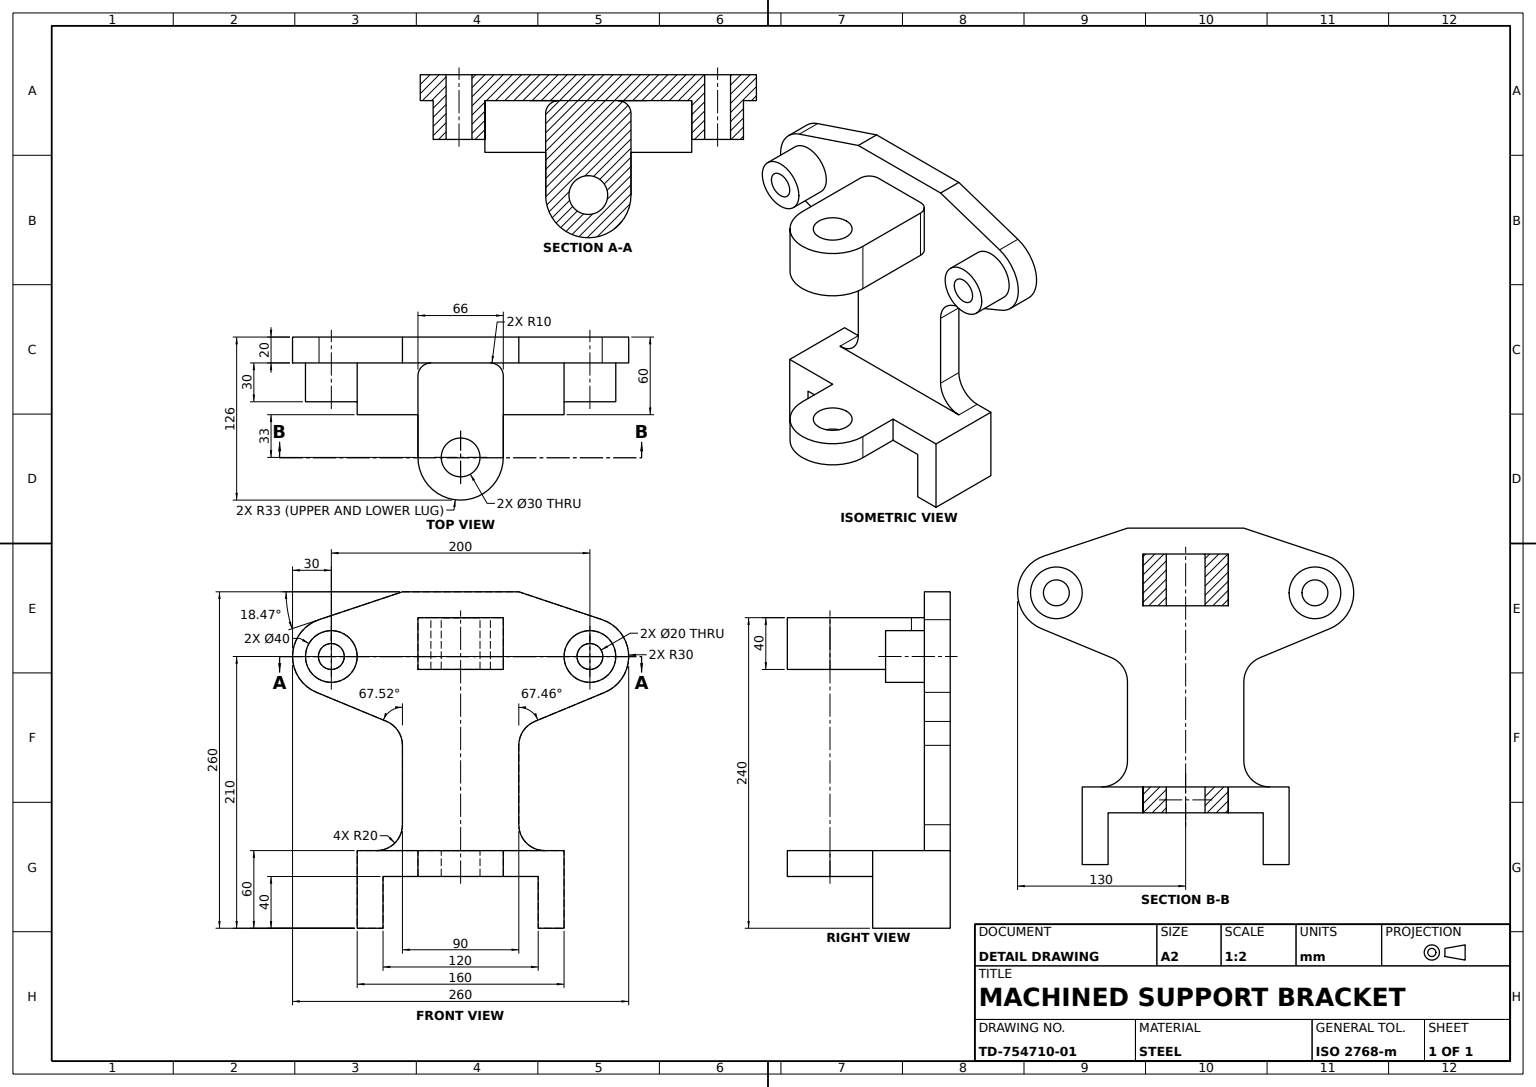
ISO-10303-21;
HEADER;
FILE_DESCRIPTION((''),'2;1');
FILE_NAME('','',(''),(''),'','','');
FILE_SCHEMA(('AUTOMOTIVE_DESIGN'));
ENDSEC;
DATA;
#1=APPLICATION_CONTEXT('');
#2=PRODUCT_CONTEXT('',#1,'mechanical');
#3=PRODUCT('','','',(#2));
#4=PRODUCT_DEFINITION_FORMATION('','',#3);
#5=PRODUCT_DEFINITION_CONTEXT('',#1,'design');
#6=PRODUCT_DEFINITION('','',#4,#5);
#7=PRODUCT_DEFINITION_SHAPE('','',#6);
#8=(LENGTH_UNIT()NAMED_UNIT(*)SI_UNIT(.MILLI.,.METRE.));
#9=(NAMED_UNIT(*)PLANE_ANGLE_UNIT()SI_UNIT($,.RADIAN.));
#10=(NAMED_UNIT(*)SI_UNIT($,.STERADIAN.)SOLID_ANGLE_UNIT());
#11=UNCERTAINTY_MEASURE_WITH_UNIT(LENGTH_MEASURE(1.E-05),#8,'distance_accuracy_value','');
#12=(GEOMETRIC_REPRESENTATION_CONTEXT(3)GLOBAL_UNCERTAINTY_ASSIGNED_CONTEXT((#11))GLOBAL_UNIT_ASSIGNED_CONTEXT((#8,#9,#10))REPRESENTATION_CONTEXT('',''));
#13=CARTESIAN_POINT('',(125.,260.,0.));
#14=VERTEX_POINT('',#13);
#15=CARTESIAN_POINT('',(35.,260.,0.));
#16=VERTEX_POINT('',#15);
#17=DIRECTION('',(-1.,0.,0.));
#18=VECTOR('',#17,1000.);
#19=LINE('',#15,#18);
#20=EDGE_CURVE('',#14,#16,#19,.T.);
#21=ORIENTED_EDGE('',*,*,#20,.T.);
#22=CARTESIAN_POINT('',(35.,260.,20.));
#23=VERTEX_POINT('',#22);
#24=DIRECTION('',(0.,0.,-1.));
#25=VECTOR('',#24,1000.);
#26=LINE('',#22,#25);
#27=EDGE_CURVE('',#23,#16,#26,.T.);
#28=ORIENTED_EDGE('',*,*,#27,.F.);
#29=CARTESIAN_POINT('',(125.,260.,20.));
#30=VERTEX_POINT('',#29);
#31=LINE('',#22,#18);
#32=EDGE_CURVE('',#30,#23,#31,.T.);
#33=ORIENTED_EDGE('',*,*,#32,.F.);
#34=LINE('',#29,#25);
#35=EDGE_CURVE('',#30,#14,#34,.T.);
#36=ORIENTED_EDGE('',*,*,#35,.T.);
#37=EDGE_LOOP('',(#21,#28,#33,#36));
#38=FACE_OUTER_BOUND('',#37,.T.);
#39=DIRECTION('',(0.,-1.,0.));
#40=AXIS2_PLACEMENT_3D('',#22,#39,#24);
#41=PLANE('',#40);
#42=ADVANCED_FACE('',(#38),#41,.F.);
#43=CARTESIAN_POINT('',(0.,60.,0.));
#44=VERTEX_POINT('',#43);
#45=CARTESIAN_POINT('',(0.,0.,0.));
#46=VERTEX_POINT('',#45);
#47=VECTOR('',#39,1000.);
#48=LINE('',#45,#47);
#49=EDGE_CURVE('',#44,#46,#48,.T.);
#50=ORIENTED_EDGE('',*,*,#49,.T.);
#51=CARTESIAN_POINT('',(0.,0.,60.));
#52=VERTEX_POINT('',#51);
#53=LINE('',#51,#25);
#54=EDGE_CURVE('',#52,#46,#53,.T.);
#55=ORIENTED_EDGE('',*,*,#54,.F.);
#56=CARTESIAN_POINT('',(0.,60.,60.));
#57=VERTEX_POINT('',#56);
#58=LINE('',#51,#47);
#59=EDGE_CURVE('',#57,#52,#58,.T.);
#60=ORIENTED_EDGE('',*,*,#59,.F.);
#61=LINE('',#56,#25);
#62=EDGE_CURVE('',#57,#44,#61,.T.);
#63=ORIENTED_EDGE('',*,*,#62,.T.);
#64=EDGE_LOOP('',(#50,#55,#60,#63));
#65=FACE_OUTER_BOUND('',#64,.T.);
#66=DIRECTION('',(1.,0.,0.));
#67=AXIS2_PLACEMENT_3D('',#51,#66,#24);
#68=PLANE('',#67);
#69=ADVANCED_FACE('',(#65),#68,.F.);
#70=CARTESIAN_POINT('',(170.,210.,50.));
#71=VERTEX_POINT('',#70);
#72=CARTESIAN_POINT('',(170.,210.,0.));
#73=VERTEX_POINT('',#72);
#74=LINE('',#70,#25);
#75=EDGE_CURVE('',#71,#73,#74,.T.);
#76=ORIENTED_EDGE('',*,*,#75,.T.);
#77=CARTESIAN_POINT('',(190.,210.,0.));
#78=VERTEX_POINT('',#77);
#79=CARTESIAN_POINT('',(180.,210.,0.));
#80=AXIS2_PLACEMENT_3D('',#79,#24,#17);
#81=CIRCLE('',#80,10.);
#82=EDGE_CURVE('',#73,#78,#81,.T.);
#83=ORIENTED_EDGE('',*,*,#82,.T.);
#84=CARTESIAN_POINT('',(190.,210.,50.));
#85=VERTEX_POINT('',#84);
#86=LINE('',#84,#25);
#87=EDGE_CURVE('',#85,#78,#86,.T.);
#88=ORIENTED_EDGE('',*,*,#87,.F.);
#89=CARTESIAN_POINT('',(180.,210.,50.));
#90=DIRECTION('',(0.,0.,1.));
#91=AXIS2_PLACEMENT_3D('',#89,#90,#66);
#92=CIRCLE('',#91,10.);
#93=EDGE_CURVE('',#85,#71,#92,.T.);
#94=ORIENTED_EDGE('',*,*,#93,.T.);
#95=EDGE_LOOP('',(#76,#83,#88,#94));
#96=FACE_OUTER_BOUND('',#95,.T.);
#97=AXIS2_PLACEMENT_3D('',#89,#24,#17);
#98=CYLINDRICAL_SURFACE('',#97,10.);
#99=ADVANCED_FACE('',(#96),#98,.F.);
#100=CARTESIAN_POINT('',(47.,60.,60.));
#101=VERTEX_POINT('',#100);
#102=CARTESIAN_POINT('',(47.,60.,93.));
#103=VERTEX_POINT('',#102);
#104=VECTOR('',#90,1000.);
#105=LINE('',#102,#104);
#106=EDGE_CURVE('',#101,#103,#105,.T.);
#107=ORIENTED_EDGE('',*,*,#106,.F.);
#108=CARTESIAN_POINT('',(47.,40.,60.));
#109=VERTEX_POINT('',#108);
#110=DIRECTION('',(0.,1.,0.));
#111=VECTOR('',#110,1000.);
#112=LINE('',#108,#111);
#113=EDGE_CURVE('',#109,#101,#112,.T.);
#114=ORIENTED_EDGE('',*,*,#113,.F.);
#115=CARTESIAN_POINT('',(47.,40.,93.));
#116=VERTEX_POINT('',#115);
#117=LINE('',#115,#104);
#118=EDGE_CURVE('',#109,#116,#117,.T.);
#119=ORIENTED_EDGE('',*,*,#118,.T.);
#120=LINE('',#115,#111);
#121=EDGE_CURVE('',#116,#103,#120,.T.);
#122=ORIENTED_EDGE('',*,*,#121,.T.);
#123=EDGE_LOOP('',(#107,#114,#119,#122));
#124=FACE_OUTER_BOUND('',#123,.T.);
#125=AXIS2_PLACEMENT_3D('',#115,#17,#90);
#126=PLANE('',#125);
#127=ADVANCED_FACE('',(#124),#126,.T.);
#128=CARTESIAN_POINT('',(80.,200.,108.));
#129=VERTEX_POINT('',#128);
#130=CARTESIAN_POINT('',(80.,200.,78.));
#131=VERTEX_POINT('',#130);
#132=CARTESIAN_POINT('',(80.,200.,93.));
#133=AXIS2_PLACEMENT_3D('',#132,#110,#90);
#134=CIRCLE('',#133,15.);
#135=EDGE_CURVE('',#129,#131,#134,.T.);
#136=ORIENTED_EDGE('',*,*,#135,.F.);
#137=CARTESIAN_POINT('',(80.,240.,108.));
#138=VERTEX_POINT('',#137);
#139=LINE('',#128,#111);
#140=EDGE_CURVE('',#129,#138,#139,.T.);
#141=ORIENTED_EDGE('',*,*,#140,.T.);
#142=CARTESIAN_POINT('',(80.,240.,78.));
#143=VERTEX_POINT('',#142);
#144=CARTESIAN_POINT('',(80.,240.,93.));
#145=AXIS2_PLACEMENT_3D('',#144,#110,#90);
#146=CIRCLE('',#145,15.);
#147=EDGE_CURVE('',#138,#143,#146,.T.);
#148=ORIENTED_EDGE('',*,*,#147,.T.);
#149=LINE('',#130,#111);
#150=EDGE_CURVE('',#131,#143,#149,.T.);
#151=ORIENTED_EDGE('',*,*,#150,.F.);
#152=EDGE_LOOP('',(#136,#141,#148,#151));
#153=FACE_OUTER_BOUND('',#152,.T.);
#154=CYLINDRICAL_SURFACE('',#133,15.);
#155=ADVANCED_FACE('',(#153),#154,.F.);
#156=CARTESIAN_POINT('',(80.,60.,78.));
#157=VERTEX_POINT('',#156);
#158=CARTESIAN_POINT('',(80.,60.,108.));
#159=VERTEX_POINT('',#158);
#160=CARTESIAN_POINT('',(80.,60.,93.));
#161=AXIS2_PLACEMENT_3D('',#160,#110,#90);
#162=CIRCLE('',#161,15.);
#163=EDGE_CURVE('',#157,#159,#162,.T.);
#164=ORIENTED_EDGE('',*,*,#163,.T.);
#165=CARTESIAN_POINT('',(80.,40.,108.));
#166=VERTEX_POINT('',#165);
#167=LINE('',#165,#111);
#168=EDGE_CURVE('',#166,#159,#167,.T.);
#169=ORIENTED_EDGE('',*,*,#168,.F.);
#170=CARTESIAN_POINT('',(80.,40.,78.));
#171=VERTEX_POINT('',#170);
#172=CARTESIAN_POINT('',(80.,40.,93.));
#173=AXIS2_PLACEMENT_3D('',#172,#110,#90);
#174=CIRCLE('',#173,15.);
#175=EDGE_CURVE('',#171,#166,#174,.T.);
#176=ORIENTED_EDGE('',*,*,#175,.F.);
#177=LINE('',#170,#111);
#178=EDGE_CURVE('',#171,#157,#177,.T.);
#179=ORIENTED_EDGE('',*,*,#178,.T.);
#180=EDGE_LOOP('',(#164,#169,#176,#179));
#181=FACE_OUTER_BOUND('',#180,.T.);
#182=CYLINDRICAL_SURFACE('',#173,15.);
#183=ADVANCED_FACE('',(#181),#182,.F.);
#184=CARTESIAN_POINT('',(22.646832,159.886795,20.));
#185=VERTEX_POINT('',#184);
#186=CARTESIAN_POINT('',(22.646832,159.886795,0.));
#187=VERTEX_POINT('',#186);
#188=LINE('',#184,#25);
#189=EDGE_CURVE('',#185,#187,#188,.T.);
#190=ORIENTED_EDGE('',*,*,#189,.T.);
#191=CARTESIAN_POINT('',(35.,141.406374,0.));
#192=VERTEX_POINT('',#191);
#193=CARTESIAN_POINT('',(15.,141.406374,0.));
#194=AXIS2_PLACEMENT_3D('',#193,#24,#66);
#195=CIRCLE('',#194,20.);
#196=EDGE_CURVE('',#187,#192,#195,.T.);
#197=ORIENTED_EDGE('',*,*,#196,.T.);
#198=CARTESIAN_POINT('',(35.,141.406374,20.));
#199=VERTEX_POINT('',#198);
#200=LINE('',#198,#25);
#201=EDGE_CURVE('',#199,#192,#200,.T.);
#202=ORIENTED_EDGE('',*,*,#201,.F.);
#203=CARTESIAN_POINT('',(15.,141.406374,20.));
#204=AXIS2_PLACEMENT_3D('',#203,#24,#66);
#205=CIRCLE('',#204,20.);
#206=EDGE_CURVE('',#185,#199,#205,.T.);
#207=ORIENTED_EDGE('',*,*,#206,.F.);
#208=EDGE_LOOP('',(#190,#197,#202,#207));
#209=FACE_OUTER_BOUND('',#208,.T.);
#210=AXIS2_PLACEMENT_3D('',#203,#24,#17);
#211=CYLINDRICAL_SURFACE('',#210,20.);
#212=ADVANCED_FACE('',(#209),#211,.F.);
#213=CARTESIAN_POINT('',(-29.504259,238.454684,20.));
#214=VERTEX_POINT('',#213);
#215=CARTESIAN_POINT('',(-29.504259,238.454684,0.));
#216=VERTEX_POINT('',#215);
#217=LINE('',#213,#25);
#218=EDGE_CURVE('',#214,#216,#217,.T.);
#219=ORIENTED_EDGE('',*,*,#218,.F.);
#220=DIRECTION('',(-0.948489482,-0.31680862,0.));
#221=VECTOR('',#220,1000.);
#222=LINE('',#22,#221);
#223=EDGE_CURVE('',#23,#214,#222,.T.);
#224=ORIENTED_EDGE('',*,*,#223,.F.);
#225=ORIENTED_EDGE('',*,*,#27,.T.);
#226=LINE('',#15,#221);
#227=EDGE_CURVE('',#16,#216,#226,.T.);
#228=ORIENTED_EDGE('',*,*,#227,.T.);
#229=EDGE_LOOP('',(#219,#224,#225,#228));
#230=FACE_OUTER_BOUND('',#229,.T.);
#231=DIRECTION('',(0.31680862,-0.948489482,0.));
#232=DIRECTION('',(0.948489482,0.31680862,0.));
#233=AXIS2_PLACEMENT_3D('',#22,#231,#232);
#234=PLANE('',#233);
#235=ADVANCED_FACE('',(#230),#234,.F.);
#236=CARTESIAN_POINT('',(160.,0.,0.));
#237=VERTEX_POINT('',#236);
#238=CARTESIAN_POINT('',(160.,60.,0.));
#239=VERTEX_POINT('',#238);
#240=LINE('',#238,#111);
#241=EDGE_CURVE('',#237,#239,#240,.T.);
#242=ORIENTED_EDGE('',*,*,#241,.T.);
#243=CARTESIAN_POINT('',(160.,60.,60.));
#244=VERTEX_POINT('',#243);
#245=LINE('',#243,#25);
#246=EDGE_CURVE('',#244,#239,#245,.T.);
#247=ORIENTED_EDGE('',*,*,#246,.F.);
#248=CARTESIAN_POINT('',(160.,0.,60.));
#249=VERTEX_POINT('',#248);
#250=LINE('',#243,#111);
#251=EDGE_CURVE('',#249,#244,#250,.T.);
#252=ORIENTED_EDGE('',*,*,#251,.F.);
#253=LINE('',#248,#25);
#254=EDGE_CURVE('',#249,#237,#253,.T.);
#255=ORIENTED_EDGE('',*,*,#254,.T.);
#256=EDGE_LOOP('',(#242,#247,#252,#255));
#257=FACE_OUTER_BOUND('',#256,.T.);
#258=AXIS2_PLACEMENT_3D('',#243,#17,#90);
#259=PLANE('',#258);
#260=ADVANCED_FACE('',(#257),#259,.F.);
#261=CARTESIAN_POINT('',(200.,210.,20.));
#262=VERTEX_POINT('',#261);
#263=CARTESIAN_POINT('',(160.,210.,20.));
#264=VERTEX_POINT('',#263);
#265=CARTESIAN_POINT('',(180.,210.,20.));
#266=AXIS2_PLACEMENT_3D('',#265,#90,#66);
#267=CIRCLE('',#266,20.);
#268=EDGE_CURVE('',#262,#264,#267,.T.);
#269=ORIENTED_EDGE('',*,*,#268,.F.);
#270=EDGE_CURVE('',#264,#262,#267,.T.);
#271=ORIENTED_EDGE('',*,*,#270,.F.);
#272=EDGE_LOOP('',(#269,#271));
#273=FACE_BOUND('',#272,.T.);
#274=CARTESIAN_POINT('',(0.,210.,20.));
#275=VERTEX_POINT('',#274);
#276=CARTESIAN_POINT('',(-40.,210.,20.));
#277=VERTEX_POINT('',#276);
#278=CARTESIAN_POINT('',(-20.,210.,20.));
#279=AXIS2_PLACEMENT_3D('',#278,#90,#66);
#280=CIRCLE('',#279,20.);
#281=EDGE_CURVE('',#275,#277,#280,.T.);
#282=ORIENTED_EDGE('',*,*,#281,.F.);
#283=EDGE_CURVE('',#277,#275,#280,.T.);
#284=ORIENTED_EDGE('',*,*,#283,.F.);
#285=EDGE_LOOP('',(#282,#284));
#286=FACE_BOUND('',#285,.T.);
#287=CARTESIAN_POINT('',(15.,60.,20.));
#288=VERTEX_POINT('',#287);
#289=CARTESIAN_POINT('',(145.,60.,20.));
#290=VERTEX_POINT('',#289);
#291=VECTOR('',#66,1000.);
#292=LINE('',#287,#291);
#293=EDGE_CURVE('',#288,#290,#292,.T.);
#294=ORIENTED_EDGE('',*,*,#293,.T.);
#295=CARTESIAN_POINT('',(125.,80.,20.));
#296=VERTEX_POINT('',#295);
#297=CARTESIAN_POINT('',(145.,80.,20.));
#298=AXIS2_PLACEMENT_3D('',#297,#24,#66);
#299=CIRCLE('',#298,20.);
#300=EDGE_CURVE('',#290,#296,#299,.T.);
#301=ORIENTED_EDGE('',*,*,#300,.T.);
#302=CARTESIAN_POINT('',(125.,141.339701,20.));
#303=VERTEX_POINT('',#302);
#304=LINE('',#302,#111);
#305=EDGE_CURVE('',#296,#303,#304,.T.);
#306=ORIENTED_EDGE('',*,*,#305,.T.);
#307=CARTESIAN_POINT('',(137.33375,159.812075,20.));
#308=VERTEX_POINT('',#307);
#309=CARTESIAN_POINT('',(145.,141.339701,20.));
#310=AXIS2_PLACEMENT_3D('',#309,#24,#17);
#311=CIRCLE('',#310,20.);
#312=EDGE_CURVE('',#303,#308,#311,.T.);
#313=ORIENTED_EDGE('',*,*,#312,.T.);
#314=CARTESIAN_POINT('',(191.499375,182.291439,20.));
#315=VERTEX_POINT('',#314);
#316=DIRECTION('',(0.923618716,0.383312493,0.));
#317=VECTOR('',#316,1000.);
#318=LINE('',#314,#317);
#319=EDGE_CURVE('',#308,#315,#318,.T.);
#320=ORIENTED_EDGE('',*,*,#319,.T.);
#321=CARTESIAN_POINT('',(189.504259,238.454684,20.));
#322=VERTEX_POINT('',#321);
#323=CIRCLE('',#266,30.);
#324=EDGE_CURVE('',#315,#322,#323,.T.);
#325=ORIENTED_EDGE('',*,*,#324,.T.);
#326=DIRECTION('',(-0.948489482,0.31680862,0.));
#327=VECTOR('',#326,1000.);
#328=LINE('',#29,#327);
#329=EDGE_CURVE('',#322,#30,#328,.T.);
#330=ORIENTED_EDGE('',*,*,#329,.T.);
#331=ORIENTED_EDGE('',*,*,#32,.T.);
#332=ORIENTED_EDGE('',*,*,#223,.T.);
#333=CARTESIAN_POINT('',(-50.,210.,20.));
#334=VERTEX_POINT('',#333);
#335=CIRCLE('',#279,30.);
#336=EDGE_CURVE('',#214,#334,#335,.T.);
#337=ORIENTED_EDGE('',*,*,#336,.T.);
#338=CARTESIAN_POINT('',(-31.470247,182.279368,20.));
#339=VERTEX_POINT('',#338);
#340=EDGE_CURVE('',#334,#339,#335,.T.);
#341=ORIENTED_EDGE('',*,*,#340,.T.);
#342=DIRECTION('',(0.92402106,-0.382341576,0.));
#343=VECTOR('',#342,1000.);
#344=LINE('',#338,#343);
#345=EDGE_CURVE('',#339,#185,#344,.T.);
#346=ORIENTED_EDGE('',*,*,#345,.T.);
#347=ORIENTED_EDGE('',*,*,#206,.T.);
#348=CARTESIAN_POINT('',(35.,80.,20.));
#349=VERTEX_POINT('',#348);
#350=LINE('',#198,#47);
#351=EDGE_CURVE('',#199,#349,#350,.T.);
#352=ORIENTED_EDGE('',*,*,#351,.T.);
#353=CARTESIAN_POINT('',(15.,80.,20.));
#354=AXIS2_PLACEMENT_3D('',#353,#24,#66);
#355=CIRCLE('',#354,20.);
#356=EDGE_CURVE('',#349,#288,#355,.T.);
#357=ORIENTED_EDGE('',*,*,#356,.T.);
#358=EDGE_LOOP('',(#294,#301,#306,#313,#320,#325,#330,#331,#332,#337,#341,#346,#347,#352,#357));
#359=FACE_OUTER_BOUND('',#358,.T.);
#360=CARTESIAN_POINT('',(103.,240.,20.));
#361=VERTEX_POINT('',#360);
#362=CARTESIAN_POINT('',(57.,240.,20.));
#363=VERTEX_POINT('',#362);
#364=LINE('',#362,#18);
#365=EDGE_CURVE('',#361,#363,#364,.T.);
#366=ORIENTED_EDGE('',*,*,#365,.F.);
#367=CARTESIAN_POINT('',(103.,200.,20.));
#368=VERTEX_POINT('',#367);
#369=LINE('',#367,#111);
#370=EDGE_CURVE('',#368,#361,#369,.T.);
#371=ORIENTED_EDGE('',*,*,#370,.F.);
#372=CARTESIAN_POINT('',(57.,200.,20.));
#373=VERTEX_POINT('',#372);
#374=LINE('',#372,#18);
#375=EDGE_CURVE('',#368,#373,#374,.T.);
#376=ORIENTED_EDGE('',*,*,#375,.T.);
#377=LINE('',#372,#111);
#378=EDGE_CURVE('',#373,#363,#377,.T.);
#379=ORIENTED_EDGE('',*,*,#378,.T.);
#380=EDGE_LOOP('',(#366,#371,#376,#379));
#381=FACE_BOUND('',#380,.T.);
#382=PLANE('',#279);
#383=ADVANCED_FACE('',(#273,#286,#359,#381),#382,.T.);
#384=CARTESIAN_POINT('',(113.,200.,93.));
#385=VERTEX_POINT('',#384);
#386=CARTESIAN_POINT('',(113.,240.,93.));
#387=VERTEX_POINT('',#386);
#388=LINE('',#384,#111);
#389=EDGE_CURVE('',#385,#387,#388,.T.);
#390=ORIENTED_EDGE('',*,*,#389,.T.);
#391=CARTESIAN_POINT('',(80.,240.,126.));
#392=VERTEX_POINT('',#391);
#393=CIRCLE('',#145,33.);
#394=EDGE_CURVE('',#392,#387,#393,.T.);
#395=ORIENTED_EDGE('',*,*,#394,.F.);
#396=CARTESIAN_POINT('',(80.,200.,126.));
#397=VERTEX_POINT('',#396);
#398=LINE('',#396,#111);
#399=EDGE_CURVE('',#397,#392,#398,.T.);
#400=ORIENTED_EDGE('',*,*,#399,.F.);
#401=CIRCLE('',#133,33.);
#402=EDGE_CURVE('',#397,#385,#401,.T.);
#403=ORIENTED_EDGE('',*,*,#402,.T.);
#404=EDGE_LOOP('',(#390,#395,#400,#403));
#405=FACE_OUTER_BOUND('',#404,.T.);
#406=CYLINDRICAL_SURFACE('',#133,33.);
#407=ADVANCED_FACE('',(#405),#406,.T.);
#408=ORIENTED_EDGE('',*,*,#370,.T.);
#409=CARTESIAN_POINT('',(113.,240.,30.));
#410=VERTEX_POINT('',#409);
#411=CARTESIAN_POINT('',(103.,240.,30.));
#412=AXIS2_PLACEMENT_3D('',#411,#110,#90);
#413=CIRCLE('',#412,10.);
#414=EDGE_CURVE('',#410,#361,#413,.T.);
#415=ORIENTED_EDGE('',*,*,#414,.F.);
#416=CARTESIAN_POINT('',(113.,200.,30.));
#417=VERTEX_POINT('',#416);
#418=LINE('',#416,#111);
#419=EDGE_CURVE('',#417,#410,#418,.T.);
#420=ORIENTED_EDGE('',*,*,#419,.F.);
#421=CARTESIAN_POINT('',(103.,200.,30.));
#422=AXIS2_PLACEMENT_3D('',#421,#110,#90);
#423=CIRCLE('',#422,10.);
#424=EDGE_CURVE('',#417,#368,#423,.T.);
#425=ORIENTED_EDGE('',*,*,#424,.T.);
#426=EDGE_LOOP('',(#408,#415,#420,#425));
#427=FACE_OUTER_BOUND('',#426,.T.);
#428=CYLINDRICAL_SURFACE('',#422,10.);
#429=ADVANCED_FACE('',(#427),#428,.T.);
#430=ORIENTED_EDGE('',*,*,#254,.F.);
#431=CARTESIAN_POINT('',(140.,0.,60.));
#432=VERTEX_POINT('',#431);
#433=LINE('',#248,#291);
#434=EDGE_CURVE('',#432,#249,#433,.T.);
#435=ORIENTED_EDGE('',*,*,#434,.F.);
#436=CARTESIAN_POINT('',(140.,0.,0.));
#437=VERTEX_POINT('',#436);
#438=LINE('',#431,#25);
#439=EDGE_CURVE('',#432,#437,#438,.T.);
#440=ORIENTED_EDGE('',*,*,#439,.T.);
#441=LINE('',#236,#291);
#442=EDGE_CURVE('',#437,#237,#441,.T.);
#443=ORIENTED_EDGE('',*,*,#442,.T.);
#444=EDGE_LOOP('',(#430,#435,#440,#443));
#445=FACE_OUTER_BOUND('',#444,.T.);
#446=AXIS2_PLACEMENT_3D('',#248,#110,#90);
#447=PLANE('',#446);
#448=ADVANCED_FACE('',(#445),#447,.F.);
#449=CARTESIAN_POINT('',(-30.,210.,50.));
#450=VERTEX_POINT('',#449);
#451=CARTESIAN_POINT('',(-30.,210.,0.));
#452=VERTEX_POINT('',#451);
#453=LINE('',#449,#25);
#454=EDGE_CURVE('',#450,#452,#453,.T.);
#455=ORIENTED_EDGE('',*,*,#454,.F.);
#456=CARTESIAN_POINT('',(-10.,210.,50.));
#457=VERTEX_POINT('',#456);
#458=CARTESIAN_POINT('',(-20.,210.,50.));
#459=AXIS2_PLACEMENT_3D('',#458,#90,#66);
#460=CIRCLE('',#459,10.);
#461=EDGE_CURVE('',#450,#457,#460,.T.);
#462=ORIENTED_EDGE('',*,*,#461,.T.);
#463=CARTESIAN_POINT('',(-10.,210.,0.));
#464=VERTEX_POINT('',#463);
#465=LINE('',#456,#25);
#466=EDGE_CURVE('',#457,#464,#465,.T.);
#467=ORIENTED_EDGE('',*,*,#466,.T.);
#468=CARTESIAN_POINT('',(-20.,210.,0.));
#469=AXIS2_PLACEMENT_3D('',#468,#24,#17);
#470=CIRCLE('',#469,10.);
#471=EDGE_CURVE('',#464,#452,#470,.T.);
#472=ORIENTED_EDGE('',*,*,#471,.T.);
#473=EDGE_LOOP('',(#455,#462,#467,#472));
#474=FACE_OUTER_BOUND('',#473,.T.);
#475=AXIS2_PLACEMENT_3D('',#458,#24,#17);
#476=CYLINDRICAL_SURFACE('',#475,10.);
#477=ADVANCED_FACE('',(#474),#476,.F.);
#478=CARTESIAN_POINT('',(125.,80.,0.));
#479=VERTEX_POINT('',#478);
#480=LINE('',#295,#25);
#481=EDGE_CURVE('',#296,#479,#480,.T.);
#482=ORIENTED_EDGE('',*,*,#481,.T.);
#483=CARTESIAN_POINT('',(125.,141.339701,0.));
#484=VERTEX_POINT('',#483);
#485=LINE('',#483,#111);
#486=EDGE_CURVE('',#479,#484,#485,.T.);
#487=ORIENTED_EDGE('',*,*,#486,.T.);
#488=LINE('',#302,#25);
#489=EDGE_CURVE('',#303,#484,#488,.T.);
#490=ORIENTED_EDGE('',*,*,#489,.F.);
#491=ORIENTED_EDGE('',*,*,#305,.F.);
#492=EDGE_LOOP('',(#482,#487,#490,#491));
#493=FACE_OUTER_BOUND('',#492,.T.);
#494=AXIS2_PLACEMENT_3D('',#302,#17,#39);
#495=PLANE('',#494);
#496=ADVANCED_FACE('',(#493),#495,.F.);
#497=LINE('',#384,#25);
#498=EDGE_CURVE('',#385,#417,#497,.T.);
#499=ORIENTED_EDGE('',*,*,#498,.T.);
#500=ORIENTED_EDGE('',*,*,#419,.T.);
#501=LINE('',#386,#25);
#502=EDGE_CURVE('',#387,#410,#501,.T.);
#503=ORIENTED_EDGE('',*,*,#502,.F.);
#504=ORIENTED_EDGE('',*,*,#389,.F.);
#505=EDGE_LOOP('',(#499,#500,#503,#504));
#506=FACE_OUTER_BOUND('',#505,.T.);
#507=AXIS2_PLACEMENT_3D('',#384,#66,#24);
#508=PLANE('',#507);
#509=ADVANCED_FACE('',(#506),#508,.T.);
#510=CARTESIAN_POINT('',(20.,0.,60.));
#511=VERTEX_POINT('',#510);
#512=CARTESIAN_POINT('',(20.,0.,0.));
#513=VERTEX_POINT('',#512);
#514=LINE('',#510,#25);
#515=EDGE_CURVE('',#511,#513,#514,.T.);
#516=ORIENTED_EDGE('',*,*,#515,.F.);
#517=LINE('',#510,#291);
#518=EDGE_CURVE('',#52,#511,#517,.T.);
#519=ORIENTED_EDGE('',*,*,#518,.F.);
#520=ORIENTED_EDGE('',*,*,#54,.T.);
#521=LINE('',#512,#291);
#522=EDGE_CURVE('',#46,#513,#521,.T.);
#523=ORIENTED_EDGE('',*,*,#522,.T.);
#524=EDGE_LOOP('',(#516,#519,#520,#523));
#525=FACE_OUTER_BOUND('',#524,.T.);
#526=AXIS2_PLACEMENT_3D('',#510,#110,#90);
#527=PLANE('',#526);
#528=ADVANCED_FACE('',(#525),#527,.F.);
#529=CARTESIAN_POINT('',(137.33375,159.812075,0.));
#530=VERTEX_POINT('',#529);
#531=LINE('',#307,#25);
#532=EDGE_CURVE('',#308,#530,#531,.T.);
#533=ORIENTED_EDGE('',*,*,#532,.T.);
#534=CARTESIAN_POINT('',(191.499375,182.291439,0.));
#535=VERTEX_POINT('',#534);
#536=LINE('',#534,#317);
#537=EDGE_CURVE('',#530,#535,#536,.T.);
#538=ORIENTED_EDGE('',*,*,#537,.T.);
#539=LINE('',#314,#25);
#540=EDGE_CURVE('',#315,#535,#539,.T.);
#541=ORIENTED_EDGE('',*,*,#540,.F.);
#542=ORIENTED_EDGE('',*,*,#319,.F.);
#543=EDGE_LOOP('',(#533,#538,#541,#542));
#544=FACE_OUTER_BOUND('',#543,.T.);
#545=DIRECTION('',(-0.383312493,0.923618716,0.));
#546=DIRECTION('',(-0.923618716,-0.383312493,0.));
#547=AXIS2_PLACEMENT_3D('',#314,#545,#546);
#548=PLANE('',#547);
#549=ADVANCED_FACE('',(#544),#548,.F.);
#550=CARTESIAN_POINT('',(140.,40.,60.));
#551=VERTEX_POINT('',#550);
#552=LINE('',#431,#47);
#553=EDGE_CURVE('',#551,#432,#552,.T.);
#554=ORIENTED_EDGE('',*,*,#553,.F.);
#555=CARTESIAN_POINT('',(140.,40.,0.));
#556=VERTEX_POINT('',#555);
#557=LINE('',#550,#25);
#558=EDGE_CURVE('',#551,#556,#557,.T.);
#559=ORIENTED_EDGE('',*,*,#558,.T.);
#560=LINE('',#436,#47);
#561=EDGE_CURVE('',#556,#437,#560,.T.);
#562=ORIENTED_EDGE('',*,*,#561,.T.);
#563=ORIENTED_EDGE('',*,*,#439,.F.);
#564=EDGE_LOOP('',(#554,#559,#562,#563));
#565=FACE_OUTER_BOUND('',#564,.T.);
#566=AXIS2_PLACEMENT_3D('',#431,#66,#24);
#567=PLANE('',#566);
#568=ADVANCED_FACE('',(#565),#567,.F.);
#569=EDGE_CURVE('',#457,#450,#460,.T.);
#570=ORIENTED_EDGE('',*,*,#569,.F.);
#571=ORIENTED_EDGE('',*,*,#461,.F.);
#572=EDGE_LOOP('',(#570,#571));
#573=FACE_BOUND('',#572,.T.);
#574=CARTESIAN_POINT('',(-40.,210.,50.));
#575=VERTEX_POINT('',#574);
#576=CARTESIAN_POINT('',(0.,210.,50.));
#577=VERTEX_POINT('',#576);
#578=CIRCLE('',#459,20.);
#579=EDGE_CURVE('',#575,#577,#578,.T.);
#580=ORIENTED_EDGE('',*,*,#579,.T.);
#581=EDGE_CURVE('',#577,#575,#578,.T.);
#582=ORIENTED_EDGE('',*,*,#581,.T.);
#583=EDGE_LOOP('',(#580,#582));
#584=FACE_OUTER_BOUND('',#583,.T.);
#585=PLANE('',#459);
#586=ADVANCED_FACE('',(#573,#584),#585,.T.);
#587=ORIENTED_EDGE('',*,*,#356,.F.);
#588=CARTESIAN_POINT('',(35.,80.,0.));
#589=VERTEX_POINT('',#588);
#590=LINE('',#348,#25);
#591=EDGE_CURVE('',#349,#589,#590,.T.);
#592=ORIENTED_EDGE('',*,*,#591,.T.);
#593=CARTESIAN_POINT('',(15.,60.,0.));
#594=VERTEX_POINT('',#593);
#595=CARTESIAN_POINT('',(15.,80.,0.));
#596=AXIS2_PLACEMENT_3D('',#595,#24,#66);
#597=CIRCLE('',#596,20.);
#598=EDGE_CURVE('',#589,#594,#597,.T.);
#599=ORIENTED_EDGE('',*,*,#598,.T.);
#600=LINE('',#287,#25);
#601=EDGE_CURVE('',#288,#594,#600,.T.);
#602=ORIENTED_EDGE('',*,*,#601,.F.);
#603=EDGE_LOOP('',(#587,#592,#599,#602));
#604=FACE_OUTER_BOUND('',#603,.T.);
#605=AXIS2_PLACEMENT_3D('',#353,#24,#17);
#606=CYLINDRICAL_SURFACE('',#605,20.);
#607=ADVANCED_FACE('',(#604),#606,.F.);
#608=EDGE_CURVE('',#143,#138,#146,.T.);
#609=ORIENTED_EDGE('',*,*,#608,.F.);
#610=ORIENTED_EDGE('',*,*,#147,.F.);
#611=EDGE_LOOP('',(#609,#610));
#612=FACE_BOUND('',#611,.T.);
#613=ORIENTED_EDGE('',*,*,#502,.T.);
#614=ORIENTED_EDGE('',*,*,#414,.T.);
#615=ORIENTED_EDGE('',*,*,#365,.T.);
#616=CARTESIAN_POINT('',(47.,240.,30.));
#617=VERTEX_POINT('',#616);
#618=CARTESIAN_POINT('',(57.,240.,30.));
#619=AXIS2_PLACEMENT_3D('',#618,#110,#90);
#620=CIRCLE('',#619,10.);
#621=EDGE_CURVE('',#363,#617,#620,.T.);
#622=ORIENTED_EDGE('',*,*,#621,.T.);
#623=CARTESIAN_POINT('',(47.,240.,93.));
#624=VERTEX_POINT('',#623);
#625=LINE('',#623,#104);
#626=EDGE_CURVE('',#617,#624,#625,.T.);
#627=ORIENTED_EDGE('',*,*,#626,.T.);
#628=EDGE_CURVE('',#624,#392,#393,.T.);
#629=ORIENTED_EDGE('',*,*,#628,.T.);
#630=ORIENTED_EDGE('',*,*,#394,.T.);
#631=EDGE_LOOP('',(#613,#614,#615,#622,#627,#629,#630));
#632=FACE_OUTER_BOUND('',#631,.T.);
#633=PLANE('',#412);
#634=ADVANCED_FACE('',(#612,#632),#633,.T.);
#635=ORIENTED_EDGE('',*,*,#434,.T.);
#636=ORIENTED_EDGE('',*,*,#251,.T.);
#637=CARTESIAN_POINT('',(113.,60.,60.));
#638=VERTEX_POINT('',#637);
#639=LINE('',#56,#18);
#640=EDGE_CURVE('',#244,#638,#639,.T.);
#641=ORIENTED_EDGE('',*,*,#640,.T.);
#642=CARTESIAN_POINT('',(113.,40.,60.));
#643=VERTEX_POINT('',#642);
#644=LINE('',#642,#111);
#645=EDGE_CURVE('',#643,#638,#644,.T.);
#646=ORIENTED_EDGE('',*,*,#645,.F.);
#647=LINE('',#550,#291);
#648=EDGE_CURVE('',#643,#551,#647,.T.);
#649=ORIENTED_EDGE('',*,*,#648,.T.);
#650=ORIENTED_EDGE('',*,*,#553,.T.);
#651=EDGE_LOOP('',(#635,#636,#641,#646,#649,#650));
#652=FACE_OUTER_BOUND('',#651,.T.);
#653=AXIS2_PLACEMENT_3D('',#51,#24,#17);
#654=PLANE('',#653);
#655=ADVANCED_FACE('',(#652),#654,.F.);
#656=CARTESIAN_POINT('',(80.,40.,126.));
#657=VERTEX_POINT('',#656);
#658=CARTESIAN_POINT('',(80.,60.,126.));
#659=VERTEX_POINT('',#658);
#660=LINE('',#656,#111);
#661=EDGE_CURVE('',#657,#659,#660,.T.);
#662=ORIENTED_EDGE('',*,*,#661,.F.);
#663=CARTESIAN_POINT('',(113.,40.,93.));
#664=VERTEX_POINT('',#663);
#665=CIRCLE('',#173,33.);
#666=EDGE_CURVE('',#657,#664,#665,.T.);
#667=ORIENTED_EDGE('',*,*,#666,.T.);
#668=CARTESIAN_POINT('',(113.,60.,93.));
#669=VERTEX_POINT('',#668);
#670=LINE('',#663,#111);
#671=EDGE_CURVE('',#664,#669,#670,.T.);
#672=ORIENTED_EDGE('',*,*,#671,.T.);
#673=CIRCLE('',#161,33.);
#674=EDGE_CURVE('',#659,#669,#673,.T.);
#675=ORIENTED_EDGE('',*,*,#674,.F.);
#676=EDGE_LOOP('',(#662,#667,#672,#675));
#677=FACE_OUTER_BOUND('',#676,.T.);
#678=CYLINDRICAL_SURFACE('',#173,33.);
#679=ADVANCED_FACE('',(#677),#678,.T.);
#680=CARTESIAN_POINT('',(47.,200.,30.));
#681=VERTEX_POINT('',#680);
#682=CARTESIAN_POINT('',(47.,200.,93.));
#683=VERTEX_POINT('',#682);
#684=LINE('',#682,#104);
#685=EDGE_CURVE('',#681,#683,#684,.T.);
#686=ORIENTED_EDGE('',*,*,#685,.T.);
#687=LINE('',#682,#111);
#688=EDGE_CURVE('',#683,#624,#687,.T.);
#689=ORIENTED_EDGE('',*,*,#688,.T.);
#690=ORIENTED_EDGE('',*,*,#626,.F.);
#691=LINE('',#680,#111);
#692=EDGE_CURVE('',#681,#617,#691,.T.);
#693=ORIENTED_EDGE('',*,*,#692,.F.);
#694=EDGE_LOOP('',(#686,#689,#690,#693));
#695=FACE_OUTER_BOUND('',#694,.T.);
#696=AXIS2_PLACEMENT_3D('',#682,#17,#90);
#697=PLANE('',#696);
#698=ADVANCED_FACE('',(#695),#697,.T.);
#699=CARTESIAN_POINT('',(20.,40.,0.));
#700=VERTEX_POINT('',#699);
#701=LINE('',#699,#111);
#702=EDGE_CURVE('',#513,#700,#701,.T.);
#703=ORIENTED_EDGE('',*,*,#702,.F.);
#704=ORIENTED_EDGE('',*,*,#522,.F.);
#705=ORIENTED_EDGE('',*,*,#49,.F.);
#706=LINE('',#43,#18);
#707=EDGE_CURVE('',#594,#44,#706,.T.);
#708=ORIENTED_EDGE('',*,*,#707,.F.);
#709=ORIENTED_EDGE('',*,*,#598,.F.);
#710=LINE('',#191,#47);
#711=EDGE_CURVE('',#192,#589,#710,.T.);
#712=ORIENTED_EDGE('',*,*,#711,.F.);
#713=ORIENTED_EDGE('',*,*,#196,.F.);
#714=CARTESIAN_POINT('',(-31.470247,182.279368,0.));
#715=VERTEX_POINT('',#714);
#716=LINE('',#714,#343);
#717=EDGE_CURVE('',#715,#187,#716,.T.);
#718=ORIENTED_EDGE('',*,*,#717,.F.);
#719=CARTESIAN_POINT('',(-50.,210.,0.));
#720=VERTEX_POINT('',#719);
#721=AXIS2_PLACEMENT_3D('',#468,#90,#66);
#722=CIRCLE('',#721,30.);
#723=EDGE_CURVE('',#720,#715,#722,.T.);
#724=ORIENTED_EDGE('',*,*,#723,.F.);
#725=EDGE_CURVE('',#216,#720,#722,.T.);
#726=ORIENTED_EDGE('',*,*,#725,.F.);
#727=ORIENTED_EDGE('',*,*,#227,.F.);
#728=ORIENTED_EDGE('',*,*,#20,.F.);
#729=CARTESIAN_POINT('',(189.504259,238.454684,0.));
#730=VERTEX_POINT('',#729);
#731=LINE('',#13,#327);
#732=EDGE_CURVE('',#730,#14,#731,.T.);
#733=ORIENTED_EDGE('',*,*,#732,.F.);
#734=AXIS2_PLACEMENT_3D('',#79,#90,#66);
#735=CIRCLE('',#734,30.);
#736=EDGE_CURVE('',#535,#730,#735,.T.);
#737=ORIENTED_EDGE('',*,*,#736,.F.);
#738=ORIENTED_EDGE('',*,*,#537,.F.);
#739=CARTESIAN_POINT('',(145.,141.339701,0.));
#740=AXIS2_PLACEMENT_3D('',#739,#24,#17);
#741=CIRCLE('',#740,20.);
#742=EDGE_CURVE('',#484,#530,#741,.T.);
#743=ORIENTED_EDGE('',*,*,#742,.F.);
#744=ORIENTED_EDGE('',*,*,#486,.F.);
#745=CARTESIAN_POINT('',(145.,60.,0.));
#746=VERTEX_POINT('',#745);
#747=CARTESIAN_POINT('',(145.,80.,0.));
#748=AXIS2_PLACEMENT_3D('',#747,#24,#66);
#749=CIRCLE('',#748,20.);
#750=EDGE_CURVE('',#746,#479,#749,.T.);
#751=ORIENTED_EDGE('',*,*,#750,.F.);
#752=EDGE_CURVE('',#239,#746,#706,.T.);
#753=ORIENTED_EDGE('',*,*,#752,.F.);
#754=ORIENTED_EDGE('',*,*,#241,.F.);
#755=ORIENTED_EDGE('',*,*,#442,.F.);
#756=ORIENTED_EDGE('',*,*,#561,.F.);
#757=LINE('',#555,#291);
#758=EDGE_CURVE('',#700,#556,#757,.T.);
#759=ORIENTED_EDGE('',*,*,#758,.F.);
#760=EDGE_LOOP('',(#703,#704,#705,#708,#709,#712,#713,#718,#724,#726,#727,#728,#733,#737,#738,#743,#744,#751,#753,#754,#755,#756,#759));
#761=FACE_OUTER_BOUND('',#760,.T.);
#762=ORIENTED_EDGE('',*,*,#471,.F.);
#763=EDGE_CURVE('',#452,#464,#470,.T.);
#764=ORIENTED_EDGE('',*,*,#763,.F.);
#765=EDGE_LOOP('',(#762,#764));
#766=FACE_BOUND('',#765,.T.);
#767=ORIENTED_EDGE('',*,*,#82,.F.);
#768=EDGE_CURVE('',#78,#73,#81,.T.);
#769=ORIENTED_EDGE('',*,*,#768,.F.);
#770=EDGE_LOOP('',(#767,#769));
#771=FACE_BOUND('',#770,.T.);
#772=AXIS2_PLACEMENT_3D('',#45,#24,#17);
#773=PLANE('',#772);
#774=ADVANCED_FACE('',(#761,#766,#771),#773,.T.);
#775=CARTESIAN_POINT('',(20.,40.,60.));
#776=VERTEX_POINT('',#775);
#777=LINE('',#775,#111);
#778=EDGE_CURVE('',#511,#776,#777,.T.);
#779=ORIENTED_EDGE('',*,*,#778,.T.);
#780=EDGE_CURVE('',#776,#109,#647,.T.);
#781=ORIENTED_EDGE('',*,*,#780,.T.);
#782=ORIENTED_EDGE('',*,*,#113,.T.);
#783=EDGE_CURVE('',#101,#57,#639,.T.);
#784=ORIENTED_EDGE('',*,*,#783,.T.);
#785=ORIENTED_EDGE('',*,*,#59,.T.);
#786=ORIENTED_EDGE('',*,*,#518,.T.);
#787=EDGE_LOOP('',(#779,#781,#782,#784,#785,#786));
#788=FACE_OUTER_BOUND('',#787,.T.);
#789=ADVANCED_FACE('',(#788),#654,.F.);
#790=ORIENTED_EDGE('',*,*,#579,.F.);
#791=LINE('',#574,#25);
#792=EDGE_CURVE('',#575,#277,#791,.T.);
#793=ORIENTED_EDGE('',*,*,#792,.T.);
#794=ORIENTED_EDGE('',*,*,#283,.T.);
#795=LINE('',#576,#25);
#796=EDGE_CURVE('',#577,#275,#795,.T.);
#797=ORIENTED_EDGE('',*,*,#796,.F.);
#798=EDGE_LOOP('',(#790,#793,#794,#797));
#799=FACE_OUTER_BOUND('',#798,.T.);
#800=CYLINDRICAL_SURFACE('',#475,20.);
#801=ADVANCED_FACE('',(#799),#800,.T.);
#802=EDGE_CURVE('',#159,#157,#162,.T.);
#803=ORIENTED_EDGE('',*,*,#802,.F.);
#804=ORIENTED_EDGE('',*,*,#163,.F.);
#805=EDGE_LOOP('',(#803,#804));
#806=FACE_BOUND('',#805,.T.);
#807=ORIENTED_EDGE('',*,*,#674,.T.);
#808=LINE('',#668,#25);
#809=EDGE_CURVE('',#669,#638,#808,.T.);
#810=ORIENTED_EDGE('',*,*,#809,.T.);
#811=ORIENTED_EDGE('',*,*,#640,.F.);
#812=ORIENTED_EDGE('',*,*,#246,.T.);
#813=ORIENTED_EDGE('',*,*,#752,.T.);
#814=LINE('',#289,#25);
#815=EDGE_CURVE('',#290,#746,#814,.T.);
#816=ORIENTED_EDGE('',*,*,#815,.F.);
#817=ORIENTED_EDGE('',*,*,#293,.F.);
#818=ORIENTED_EDGE('',*,*,#601,.T.);
#819=ORIENTED_EDGE('',*,*,#707,.T.);
#820=ORIENTED_EDGE('',*,*,#62,.F.);
#821=ORIENTED_EDGE('',*,*,#783,.F.);
#822=ORIENTED_EDGE('',*,*,#106,.T.);
#823=EDGE_CURVE('',#103,#659,#673,.T.);
#824=ORIENTED_EDGE('',*,*,#823,.T.);
#825=EDGE_LOOP('',(#807,#810,#811,#812,#813,#816,#817,#818,#819,#820,#821,#822,#824));
#826=FACE_OUTER_BOUND('',#825,.T.);
#827=AXIS2_PLACEMENT_3D('',#56,#39,#24);
#828=PLANE('',#827);
#829=ADVANCED_FACE('',(#806,#826),#828,.F.);
#830=LINE('',#321,#25);
#831=EDGE_CURVE('',#322,#730,#830,.T.);
#832=ORIENTED_EDGE('',*,*,#831,.T.);
#833=ORIENTED_EDGE('',*,*,#732,.T.);
#834=ORIENTED_EDGE('',*,*,#35,.F.);
#835=ORIENTED_EDGE('',*,*,#329,.F.);
#836=EDGE_LOOP('',(#832,#833,#834,#835));
#837=FACE_OUTER_BOUND('',#836,.T.);
#838=DIRECTION('',(-0.31680862,-0.948489482,0.));
#839=DIRECTION('',(0.948489482,-0.31680862,0.));
#840=AXIS2_PLACEMENT_3D('',#29,#838,#839);
#841=PLANE('',#840);
#842=ADVANCED_FACE('',(#837),#841,.F.);
#843=CARTESIAN_POINT('',(160.,210.,50.));
#844=VERTEX_POINT('',#843);
#845=CARTESIAN_POINT('',(200.,210.,50.));
#846=VERTEX_POINT('',#845);
#847=CIRCLE('',#91,20.);
#848=EDGE_CURVE('',#844,#846,#847,.T.);
#849=ORIENTED_EDGE('',*,*,#848,.F.);
#850=LINE('',#843,#25);
#851=EDGE_CURVE('',#844,#264,#850,.T.);
#852=ORIENTED_EDGE('',*,*,#851,.T.);
#853=ORIENTED_EDGE('',*,*,#270,.T.);
#854=LINE('',#845,#25);
#855=EDGE_CURVE('',#846,#262,#854,.T.);
#856=ORIENTED_EDGE('',*,*,#855,.F.);
#857=EDGE_LOOP('',(#849,#852,#853,#856));
#858=FACE_OUTER_BOUND('',#857,.T.);
#859=CYLINDRICAL_SURFACE('',#97,20.);
#860=ADVANCED_FACE('',(#858),#859,.T.);
#861=LINE('',#333,#25);
#862=EDGE_CURVE('',#334,#720,#861,.T.);
#863=ORIENTED_EDGE('',*,*,#862,.F.);
#864=ORIENTED_EDGE('',*,*,#336,.F.);
#865=ORIENTED_EDGE('',*,*,#218,.T.);
#866=ORIENTED_EDGE('',*,*,#725,.T.);
#867=EDGE_LOOP('',(#863,#864,#865,#866));
#868=FACE_OUTER_BOUND('',#867,.T.);
#869=AXIS2_PLACEMENT_3D('',#278,#24,#17);
#870=CYLINDRICAL_SURFACE('',#869,30.);
#871=ADVANCED_FACE('',(#868),#870,.T.);
#872=ORIENTED_EDGE('',*,*,#178,.F.);
#873=EDGE_CURVE('',#166,#171,#174,.T.);
#874=ORIENTED_EDGE('',*,*,#873,.F.);
#875=ORIENTED_EDGE('',*,*,#168,.T.);
#876=ORIENTED_EDGE('',*,*,#802,.T.);
#877=EDGE_LOOP('',(#872,#874,#875,#876));
#878=FACE_OUTER_BOUND('',#877,.T.);
#879=ADVANCED_FACE('',(#878),#182,.F.);
#880=ORIENTED_EDGE('',*,*,#809,.F.);
#881=ORIENTED_EDGE('',*,*,#671,.F.);
#882=LINE('',#663,#25);
#883=EDGE_CURVE('',#664,#643,#882,.T.);
#884=ORIENTED_EDGE('',*,*,#883,.T.);
#885=ORIENTED_EDGE('',*,*,#645,.T.);
#886=EDGE_LOOP('',(#880,#881,#884,#885));
#887=FACE_OUTER_BOUND('',#886,.T.);
#888=AXIS2_PLACEMENT_3D('',#663,#66,#24);
#889=PLANE('',#888);
#890=ADVANCED_FACE('',(#887),#889,.T.);
#891=LINE('',#775,#25);
#892=EDGE_CURVE('',#776,#700,#891,.T.);
#893=ORIENTED_EDGE('',*,*,#892,.T.);
#894=ORIENTED_EDGE('',*,*,#758,.T.);
#895=ORIENTED_EDGE('',*,*,#558,.F.);
#896=ORIENTED_EDGE('',*,*,#648,.F.);
#897=ORIENTED_EDGE('',*,*,#883,.F.);
#898=ORIENTED_EDGE('',*,*,#666,.F.);
#899=EDGE_CURVE('',#116,#657,#665,.T.);
#900=ORIENTED_EDGE('',*,*,#899,.F.);
#901=ORIENTED_EDGE('',*,*,#118,.F.);
#902=ORIENTED_EDGE('',*,*,#780,.F.);
#903=EDGE_LOOP('',(#893,#894,#895,#896,#897,#898,#900,#901,#902));
#904=FACE_OUTER_BOUND('',#903,.T.);
#905=ORIENTED_EDGE('',*,*,#873,.T.);
#906=ORIENTED_EDGE('',*,*,#175,.T.);
#907=EDGE_LOOP('',(#905,#906));
#908=FACE_BOUND('',#907,.T.);
#909=AXIS2_PLACEMENT_3D('',#550,#110,#90);
#910=PLANE('',#909);
#911=ADVANCED_FACE('',(#904,#908),#910,.F.);
#912=ORIENTED_EDGE('',*,*,#862,.T.);
#913=ORIENTED_EDGE('',*,*,#723,.T.);
#914=LINE('',#338,#25);
#915=EDGE_CURVE('',#339,#715,#914,.T.);
#916=ORIENTED_EDGE('',*,*,#915,.F.);
#917=ORIENTED_EDGE('',*,*,#340,.F.);
#918=EDGE_LOOP('',(#912,#913,#916,#917));
#919=FACE_OUTER_BOUND('',#918,.T.);
#920=ADVANCED_FACE('',(#919),#870,.T.);
#921=ORIENTED_EDGE('',*,*,#581,.F.);
#922=ORIENTED_EDGE('',*,*,#796,.T.);
#923=ORIENTED_EDGE('',*,*,#281,.T.);
#924=ORIENTED_EDGE('',*,*,#792,.F.);
#925=EDGE_LOOP('',(#921,#922,#923,#924));
#926=FACE_OUTER_BOUND('',#925,.T.);
#927=ADVANCED_FACE('',(#926),#800,.T.);
#928=ORIENTED_EDGE('',*,*,#189,.F.);
#929=ORIENTED_EDGE('',*,*,#345,.F.);
#930=ORIENTED_EDGE('',*,*,#915,.T.);
#931=ORIENTED_EDGE('',*,*,#717,.T.);
#932=EDGE_LOOP('',(#928,#929,#930,#931));
#933=FACE_OUTER_BOUND('',#932,.T.);
#934=DIRECTION('',(0.382341576,0.92402106,0.));
#935=DIRECTION('',(-0.92402106,0.382341576,0.));
#936=AXIS2_PLACEMENT_3D('',#338,#934,#935);
#937=PLANE('',#936);
#938=ADVANCED_FACE('',(#933),#937,.F.);
#939=ORIENTED_EDGE('',*,*,#351,.F.);
#940=ORIENTED_EDGE('',*,*,#201,.T.);
#941=ORIENTED_EDGE('',*,*,#711,.T.);
#942=ORIENTED_EDGE('',*,*,#591,.F.);
#943=EDGE_LOOP('',(#939,#940,#941,#942));
#944=FACE_OUTER_BOUND('',#943,.T.);
#945=AXIS2_PLACEMENT_3D('',#198,#66,#24);
#946=PLANE('',#945);
#947=ADVANCED_FACE('',(#944),#946,.F.);
#948=ORIENTED_EDGE('',*,*,#736,.T.);
#949=ORIENTED_EDGE('',*,*,#831,.F.);
#950=ORIENTED_EDGE('',*,*,#324,.F.);
#951=ORIENTED_EDGE('',*,*,#540,.T.);
#952=EDGE_LOOP('',(#948,#949,#950,#951));
#953=FACE_OUTER_BOUND('',#952,.T.);
#954=AXIS2_PLACEMENT_3D('',#265,#24,#17);
#955=CYLINDRICAL_SURFACE('',#954,30.);
#956=ADVANCED_FACE('',(#953),#955,.T.);
#957=ORIENTED_EDGE('',*,*,#899,.T.);
#958=ORIENTED_EDGE('',*,*,#661,.T.);
#959=ORIENTED_EDGE('',*,*,#823,.F.);
#960=ORIENTED_EDGE('',*,*,#121,.F.);
#961=EDGE_LOOP('',(#957,#958,#959,#960));
#962=FACE_OUTER_BOUND('',#961,.T.);
#963=ADVANCED_FACE('',(#962),#678,.T.);
#964=ORIENTED_EDGE('',*,*,#692,.T.);
#965=ORIENTED_EDGE('',*,*,#621,.F.);
#966=ORIENTED_EDGE('',*,*,#378,.F.);
#967=CARTESIAN_POINT('',(57.,200.,30.));
#968=AXIS2_PLACEMENT_3D('',#967,#110,#90);
#969=CIRCLE('',#968,10.);
#970=EDGE_CURVE('',#373,#681,#969,.T.);
#971=ORIENTED_EDGE('',*,*,#970,.T.);
#972=EDGE_LOOP('',(#964,#965,#966,#971));
#973=FACE_OUTER_BOUND('',#972,.T.);
#974=CYLINDRICAL_SURFACE('',#968,10.);
#975=ADVANCED_FACE('',(#973),#974,.T.);
#976=EDGE_CURVE('',#131,#129,#134,.T.);
#977=ORIENTED_EDGE('',*,*,#976,.T.);
#978=ORIENTED_EDGE('',*,*,#135,.T.);
#979=EDGE_LOOP('',(#977,#978));
#980=FACE_BOUND('',#979,.T.);
#981=ORIENTED_EDGE('',*,*,#375,.F.);
#982=ORIENTED_EDGE('',*,*,#424,.F.);
#983=ORIENTED_EDGE('',*,*,#498,.F.);
#984=ORIENTED_EDGE('',*,*,#402,.F.);
#985=EDGE_CURVE('',#683,#397,#401,.T.);
#986=ORIENTED_EDGE('',*,*,#985,.F.);
#987=ORIENTED_EDGE('',*,*,#685,.F.);
#988=ORIENTED_EDGE('',*,*,#970,.F.);
#989=EDGE_LOOP('',(#981,#982,#983,#984,#986,#987,#988));
#990=FACE_OUTER_BOUND('',#989,.T.);
#991=PLANE('',#422);
#992=ADVANCED_FACE('',(#980,#990),#991,.F.);
#993=ORIENTED_EDGE('',*,*,#489,.T.);
#994=ORIENTED_EDGE('',*,*,#742,.T.);
#995=ORIENTED_EDGE('',*,*,#532,.F.);
#996=ORIENTED_EDGE('',*,*,#312,.F.);
#997=EDGE_LOOP('',(#993,#994,#995,#996));
#998=FACE_OUTER_BOUND('',#997,.T.);
#999=CYLINDRICAL_SURFACE('',#310,20.);
#1000=ADVANCED_FACE('',(#998),#999,.F.);
#1001=ORIENTED_EDGE('',*,*,#93,.F.);
#1002=EDGE_CURVE('',#71,#85,#92,.T.);
#1003=ORIENTED_EDGE('',*,*,#1002,.F.);
#1004=EDGE_LOOP('',(#1001,#1003));
#1005=FACE_BOUND('',#1004,.T.);
#1006=EDGE_CURVE('',#846,#844,#847,.T.);
#1007=ORIENTED_EDGE('',*,*,#1006,.T.);
#1008=ORIENTED_EDGE('',*,*,#848,.T.);
#1009=EDGE_LOOP('',(#1007,#1008));
#1010=FACE_OUTER_BOUND('',#1009,.T.);
#1011=PLANE('',#91);
#1012=ADVANCED_FACE('',(#1005,#1010),#1011,.T.);
#1013=ORIENTED_EDGE('',*,*,#481,.F.);
#1014=ORIENTED_EDGE('',*,*,#300,.F.);
#1015=ORIENTED_EDGE('',*,*,#815,.T.);
#1016=ORIENTED_EDGE('',*,*,#750,.T.);
#1017=EDGE_LOOP('',(#1013,#1014,#1015,#1016));
#1018=FACE_OUTER_BOUND('',#1017,.T.);
#1019=AXIS2_PLACEMENT_3D('',#297,#24,#17);
#1020=CYLINDRICAL_SURFACE('',#1019,20.);
#1021=ADVANCED_FACE('',(#1018),#1020,.F.);
#1022=ORIENTED_EDGE('',*,*,#608,.T.);
#1023=ORIENTED_EDGE('',*,*,#140,.F.);
#1024=ORIENTED_EDGE('',*,*,#976,.F.);
#1025=ORIENTED_EDGE('',*,*,#150,.T.);
#1026=EDGE_LOOP('',(#1022,#1023,#1024,#1025));
#1027=FACE_OUTER_BOUND('',#1026,.T.);
#1028=ADVANCED_FACE('',(#1027),#154,.F.);
#1029=ORIENTED_EDGE('',*,*,#75,.F.);
#1030=ORIENTED_EDGE('',*,*,#1002,.T.);
#1031=ORIENTED_EDGE('',*,*,#87,.T.);
#1032=ORIENTED_EDGE('',*,*,#768,.T.);
#1033=EDGE_LOOP('',(#1029,#1030,#1031,#1032));
#1034=FACE_OUTER_BOUND('',#1033,.T.);
#1035=ADVANCED_FACE('',(#1034),#98,.F.);
#1036=ORIENTED_EDGE('',*,*,#778,.F.);
#1037=ORIENTED_EDGE('',*,*,#515,.T.);
#1038=ORIENTED_EDGE('',*,*,#702,.T.);
#1039=ORIENTED_EDGE('',*,*,#892,.F.);
#1040=EDGE_LOOP('',(#1036,#1037,#1038,#1039));
#1041=FACE_OUTER_BOUND('',#1040,.T.);
#1042=AXIS2_PLACEMENT_3D('',#775,#17,#90);
#1043=PLANE('',#1042);
#1044=ADVANCED_FACE('',(#1041),#1043,.F.);
#1045=ORIENTED_EDGE('',*,*,#1006,.F.);
#1046=ORIENTED_EDGE('',*,*,#855,.T.);
#1047=ORIENTED_EDGE('',*,*,#268,.T.);
#1048=ORIENTED_EDGE('',*,*,#851,.F.);
#1049=EDGE_LOOP('',(#1045,#1046,#1047,#1048));
#1050=FACE_OUTER_BOUND('',#1049,.T.);
#1051=ADVANCED_FACE('',(#1050),#859,.T.);
#1052=ORIENTED_EDGE('',*,*,#763,.T.);
#1053=ORIENTED_EDGE('',*,*,#466,.F.);
#1054=ORIENTED_EDGE('',*,*,#569,.T.);
#1055=ORIENTED_EDGE('',*,*,#454,.T.);
#1056=EDGE_LOOP('',(#1052,#1053,#1054,#1055));
#1057=FACE_OUTER_BOUND('',#1056,.T.);
#1058=ADVANCED_FACE('',(#1057),#476,.F.);
#1059=ORIENTED_EDGE('',*,*,#688,.F.);
#1060=ORIENTED_EDGE('',*,*,#985,.T.);
#1061=ORIENTED_EDGE('',*,*,#399,.T.);
#1062=ORIENTED_EDGE('',*,*,#628,.F.);
#1063=EDGE_LOOP('',(#1059,#1060,#1061,#1062));
#1064=FACE_OUTER_BOUND('',#1063,.T.);
#1065=ADVANCED_FACE('',(#1064),#406,.T.);
#1066=CLOSED_SHELL('',(#42,#69,#99,#127,#155,#183,#212,#235,#260,#383,#407,#429,#448,#477,#496,#509,#528,#549,#568,#586,#607,#634,#655,#679,#698,#774,#789,#801,#829,#842,#860,#871,#879,#890,#911,#920,#927,#938,#947,#956,#963,#975,#992,#1000,#1012,#1021,#1028,#1035,#1044,#1051,#1058,#1065));
#1067=MANIFOLD_SOLID_BREP('',#1066);
#1068=ADVANCED_BREP_SHAPE_REPRESENTATION('',(#1067),#12);
#1069=SHAPE_DEFINITION_REPRESENTATION(#7,#1068);
ENDSEC;
END-ISO-10303-21;
